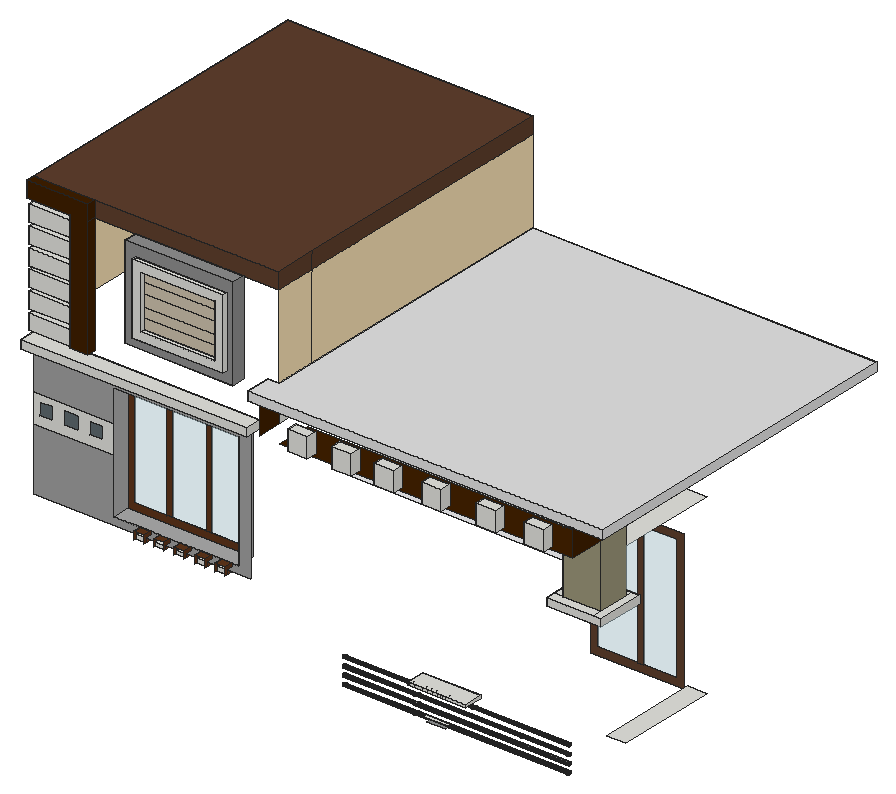
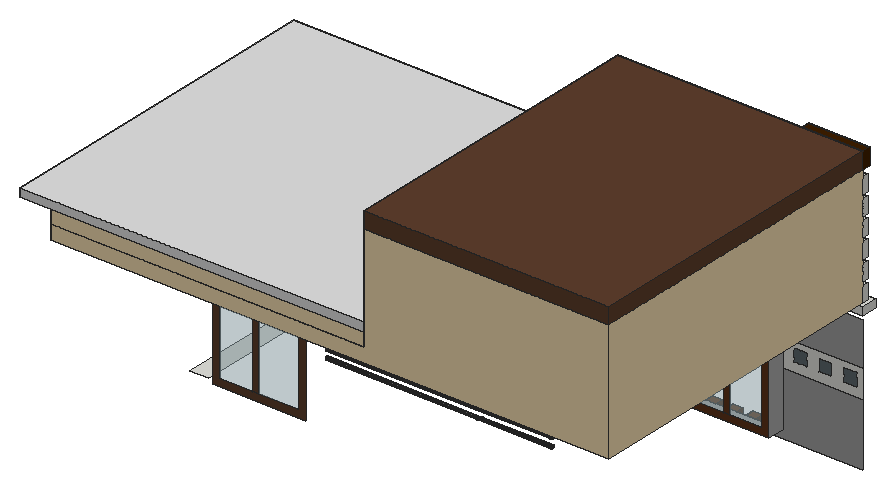
# SketchUp Ruby script. Lengths in inches.
U = 1.inch
M = Sketchup.active_model
def pt(a) = Geom::Point3d.new(a.map { |v| v * U })
def face(e, loops, mat)
  f = e.add_face(loops[0].map { |a| pt(a) })
  loops[1..].each { |l| e.add_face(l.map { |a| pt(a) }).erase! }
  f.material = f.back_material = mat if mat
  f
end
# faces: each face lists its corners as indices into pts; further lists are holes
def faces(e, pts, list, mat = nil) = list.each { |f| face(e, (f[0].is_a?(Array) ? f : [f]).map { |l| l.map { |i| pts[i] } }, mat) }
# xy, xz, yz: faces in a plane at the given z, y or x. An outline is a flat list of corners, or four numbers for a rectangle; further outlines are holes
def ring(l) = l.size == 4 ? [[l[0], l[1]], [l[2], l[1]], [l[2], l[3]], [l[0], l[3]]] : l.each_slice(2).to_a
def flat(e, list, mat, &to3) = list.each { |f| face(e, (f[0].is_a?(Array) ? f : [f]).map { |l| ring(l).map { |u, v| to3.(u, v) } }, mat) }
def xy(e, z, list, mat = nil) = flat(e, list, mat) { |x, y| [x, y, z] }
def xz(e, y, list, mat = nil) = flat(e, list, mat) { |x, z| [x, y, z] }
def yz(e, x, list, mat = nil) = flat(e, list, mat) { |y, z| [x, y, z] }
def lines(e, pts, list) = list.each { |a, b| e.add_line(pt(pts[a]), pt(pts[b])) }
# prism: a flat outline (further loops are holes) pulled along v
def prism(e, loops, v, mat = nil)
  f = face(e, loops, mat); d = Geom::Vector3d.new(v.map { |x| x * U })
  f.pushpull(f.normal.samedirection?(d) ? d.length : -d.length)
end
def box(e, o, s, mat = nil) = prism(e, [[o, [o[0] + s[0], o[1], o[2]], [o[0] + s[0], o[1] + s[1], o[2]], [o[0], o[1] + s[1], o[2]]]], [0, 0, s[2]], mat)
def at(x, y, z, deg = 0) = Geom::Transformation.translation(pt([x, y, z])) * Geom::Transformation.rotation(ORIGIN, Z_AXIS, deg.degrees)
def axes(o, x, y, z) = Geom::Transformation.new([*x, 0, *y, 0, *z, 0, *pt(o).to_a, 1])
def part(name) = M.definitions.add(name)
# library, detail: a bought-in or finely detailed component or shape, given as its bounding box
def library(name, o, s) = part(name).tap { |d| box(d.entities, o, s) }
def detail(e, o, s) = box(e.add_group.entities, o, s)
def put(e, d, t, mat = nil) = e.add_instance(d, t).tap { |i| i.material = mat if mat }
def group(e, t, mat = nil) = e.add_group.tap { |g| g.transformation = t; g.material = mat if mat }.entities
root = M.entities
M.materials.add("[0034_Wheat]").color = [245, 222, 179]
M.materials.add("[0133_Gray]").color = [128, 128, 128]
M.materials.add("[Blacktop Old 02]").color = [143, 145, 145]
M.materials.add("[Blinds Vertical Pattern]").color = [232, 232, 234]
M.materials.add("[Blinds Vertical Stripe Gray]2").color = [160, 160, 160]
M.materials.add("[Color C08]").color = [63, 31, 0]
M.materials.add("[Color M01]").color = [226, 226, 226]
M.materials.add("[Color M03]").color = [170, 170, 170]
M.materials.add("[Color M04]").color = [142, 142, 142]
M.materials.add("[Formica Speckled Grey]").color = [94, 105, 111]
M.materials.add("[Siding Rusty Metal]").color = [206, 195, 174]
M.materials.add("[Stone Coursed Rough]").color = [155, 150, 122]
M.materials.add("[Translucent Glass Safety]").color = [204, 235, 244]
M.materials["[Translucent Glass Safety]"].alpha = 0.5
M.materials.add("[Wood Cherry Original]").color = [94, 53, 26]
M.materials.add("[Wood Veneer 02]").color = [94, 63, 45]
prism(root,[[[243.46,225.17,177],[243.46,231.66,177],[243.46,231.66,178.25],[243.46,223.79,178.25],[243.46,223.79,177]]],[-24.18,0,0])
box(root,[66.16,213.82,253.05],[94.05,7.06,3.35])
box(root,[183.39,206.29,259.25],[8.18,4.44,8.19])
box(root,[281.76,206.29,259.25],[8.19,4.44,8.19])
box(root,[201.64,206.29,259.25],[8.18,4.44,8.19])
box(root,[261.82,206.29,259.25],[8.19,4.44,8.19])
box(root,[219.32,206.29,259.25],[8.19,4.44,8.19])
box(root,[239.14,206.29,259.25],[8.18,4.44,8.19])
xy(root,166.24,[[227.37,223.92,234.96,225.17]],"[Blacktop Old 02]")
xy(root,167.57,[[226.04,223.92,236.29,225.17]])
xy(root,171.3125,[[263.52,227.49,263.76,227.52,263.99,227.61,264.18,227.76,264.33,227.96,264.43,228.18,264.46,228.42,264.43,228.67,264.33,228.89,264.18,229.09,263.99,229.24,263.76,229.33,263.52,229.36,263.28,229.33,263.05,229.24,262.86,229.09,262.71,228.89,262.61,228.67,262.58,228.42,262.61,228.18,262.71,227.96,262.86,227.76,263.05,227.61,263.28,227.52]])
xy(root,171.43,[[203.52,227.49,203.76,227.52,203.99,227.61,204.18,227.76,204.29,227.9,202.75,227.9,202.86,227.76,203.05,227.61,203.28,227.52],[202.75,227.9,204.29,227.9,204.33,227.96,204.43,228.18,204.46,228.42,204.43,228.67,204.33,228.89,204.18,229.09,204.1,229.15,202.94,229.15,202.86,229.09,202.71,228.89,202.61,228.67,202.58,228.42,202.61,228.18,202.71,227.96],[202.94,229.15,204.1,229.15,203.99,229.24,203.76,229.33,203.52,229.36,203.28,229.33,203.05,229.24]])
xy(root,177,[[290.82,238.17,298.6,280.2]])
xy(root,195.78,[[110.6,218.15,114.76,220.88],[118.6,218.375,122.76,220.88],[127.16,218.375,131.32,220.88],[135.85,218.375,140.01,220.88],[144.35,218.375,148.51,220.88]],"[Wood Cherry Original]")
xy(root,197.57,[[110.6,218.15,114.76,220.88],[118.6,218.375,122.76,220.88],[127.16,218.375,131.32,220.88],[135.85,218.375,140.01,220.88],[144.35,218.375,148.51,220.88]])
xy(root,199.07,[[99.41,220.88,151.47,228.13]],"[Color M03]")
xy(root,199.07,[[110.6,217.51,114.76,220.88],[118.6,217.51,122.76,220.88],[127.16,217.51,131.32,220.88],[135.85,217.51,140.01,220.88],[144.35,217.51,148.51,220.88]],"[Wood Cherry Original]")
xy(root,228.8125,[[279.22,221.17,298.6,225.17],[298.6,221.17,301.97,241.23],[279.22,225.17,283.04,241.23],[283.04,225.17,298.6,238.17],[283.04,238.17,298.6,241.23]])
xy(root,231.84,[[279.22,221.17,298.6,225.17],[298.6,221.17,301.97,241.23],[279.22,225.17,283.04,241.23],[283.04,225.17,298.6,238.17],[283.04,238.17,298.6,241.23]])
xy(root,245.5,[[189.02,225.17,283.04,238.17]],"[Blinds Vertical Pattern]")
xy(root,246.88,[[99.41,220.88,151.47,228.13]],"[Color M03]")
xy(root,250.375,[[189.02,238.17,298.6,280.2]])
xy(root,257.875,[[283.04,225.17,298.6,238.17]])
xy(root,257.875,[[176.75,210.73,298.6,225.17]],"[Color C08]")
xy(root,263.875,[[168.19,238.17,298.6,352.92]])
xy(root,264.49,[[66.16,218.38,84.125,220.88]])
xy(root,269.1875,[[108.42,215.57,153.36,220.88]],"[Color M04]")
xy(root,269.25,[[163.51,210.73,168.19,220.88],[168.19,210.73,298.6,352.92],[298.6,210.73,311.1,352.92]])
xy(root,272.55,[[66.16,218.38,84.125,220.88]])
xy(root,272.9375,[[163.51,210.73,311.1,210.73,311.1,352.92,168.19,352.92,168.19,220.88,163.51,220.88]],"[Color M01]")
xy(root,273.55,[[112.8,213.76,150.62,215.57]])
xy(root,277.01,[[116.26,213.76,147.16,215.57]])
xy(root,280.61,[[66.16,218.38,84.125,220.88]])
xy(root,288.67,[[66.16,218.38,84.125,220.88]])
xy(root,296.74,[[66.16,218.38,84.125,220.88]])
xy(root,299.28,[[116.26,213.76,147.16,215.57]])
xy(root,302.74,[[112.8,213.76,150.62,215.57]])
xy(root,304.97,[[66.16,218.38,84.125,220.88]])
xy(root,307.625,[[66.16,217.32,84.125,220.88]])
xy(root,307.625,[[108.42,215.57,153.36,220.88]],"[Color M04]")
xy(root,314.5,[[66.16,217.32,91.59,220.88]],"[Color C08]")
xy(root,314.5,[[66.16,220.88,168.19,352.92]],"[Wood Veneer 02]")
xz(root,210.73,[[163.51,269.25,311.1,272.9375]],"[Color M01]")
xz(root,213.76,[[[112.8,273.55,150.62,302.74],[116.26,277.01,147.16,299.28]]])
xz(root,215.57,[[[112.8,273.55,150.62,302.74],[116.26,277.01,147.16,299.28]]])
xz(root,215.57,[[[108.42,269.1875,153.36,307.625],[112.8,273.55,150.62,302.74]]],"[Color M04]")
xz(root,215.57,[[116.26,277.01,147.16,281.22],[116.26,281.22,147.16,285.4375],[116.26,285.4375,147.16,290.39],[116.26,290.39,147.16,294.66],[116.26,294.66,147.16,299.28]],"[Siding Rusty Metal]")
xz(root,217.32,[[84.125,258.01,91.59,258.0625,91.59,314.5,66.16,314.5,66.16,307.625,84.125,307.625]],"[Color C08]")
xz(root,218.15,[[110.6,195.78,114.76,197.57]])
xz(root,218.375,[[118.6,195.78,122.76,197.57],[127.16,195.78,131.32,197.57],[135.85,195.78,140.01,197.57],[144.35,195.78,148.51,197.57]])
xz(root,218.38,[[66.16,257.875,84.125,258.01,84.125,264.49,66.16,264.49],[66.16,265.9375,84.125,266.07,84.125,272.55,66.16,272.55],[66.16,274,84.125,274.13,84.125,280.61,66.16,280.61],[66.16,282.0625,84.125,282.19,84.125,288.67,66.16,288.67],[66.16,290.125,84.125,290.26,84.125,296.74,66.16,296.74],
  [66.16,298.36,84.125,298.49,84.125,304.97,66.16,304.97]])
xz(root,220.88,[[110.6,197.57,114.76,199.07],[118.6,197.57,122.76,199.07],[127.16,197.57,131.32,199.07],[135.85,197.57,140.01,199.07],[144.35,197.57,148.51,199.07],
  [[66.16,221.98,99.41,233.67],[68.73,225.92,73.98,231.17],[89.61,225.92,94.86,231.17],[79.11,225.92,84.36,231.17]],[66.16,257.875,66.16,264.49,84.125,264.49,84.125,258.01],[84.125,258.01,84.125,307.625,66.16,307.625,66.16,314.5,91.59,314.5,91.59,258.0625],[66.16,265.9375,66.16,272.55,84.125,272.55,84.125,266.07],[108.42,269.1875,153.36,307.625],
  [163.51,269.25,168.19,272.9375],[66.16,274,66.16,280.61,84.125,280.61,84.125,274.13],[66.16,282.0625,66.16,288.67,84.125,288.67,84.125,282.19],[66.16,290.125,66.16,296.74,84.125,296.74,84.125,290.26],[66.16,298.36,66.16,304.97,84.125,304.97,84.125,298.49]])
xz(root,220.88,[[66.16,195.78,156.36,195.78,156.36,251.53,66.16,251.53,66.16,233.67,99.41,233.67,99.41,246.88,151.47,246.88,151.47,199.07,148.51,199.07,148.51,197.57,144.35,197.57,144.35,199.07,140.01,199.07,140.01,197.57,135.85,197.57,135.85,199.07,131.32,199.07,131.32,197.57,127.16,197.57,127.16,199.07,122.76,199.07,122.76,197.57,118.6,197.57,118.6,199.07,114.76,199.07,114.76,197.57,110.6,197.57,110.6,199.07,99.41,199.07,99.41,221.98,66.16,221.98]],"[Blinds Vertical Stripe Gray]2")
xz(root,220.88,[[66.16,264.49,84.125,264.49,84.125,266.07,66.16,265.9375],[66.16,272.55,84.125,272.55,84.125,274.13,66.16,274],[66.16,280.61,84.125,280.61,84.125,282.19,66.16,282.0625],[66.16,288.67,84.125,288.67,84.125,290.26,66.16,290.125],[66.16,296.74,84.125,296.74,84.125,298.49,66.16,298.36],
  [66.16,304.97,84.125,307.625]],"[Color C08]")
xz(root,220.88,[[68.73,225.92,73.98,231.17],[79.11,225.92,84.36,231.17],[89.61,225.92,94.86,231.17]],"[Formica Speckled Grey]")
xz(root,220.88,[[91.59,307.625,168.19,314.5]],"[Wood Veneer 02]")
xz(root,221.17,[[279.22,228.8125,301.97,231.84]])
xz(root,225.17,[[283.04,231.84,298.6,257.875]],"[Stone Coursed Rough]")
xz(root,228.13,[[102.28,201.94,115.85,244.01],[118.18,201.94,132.16,244.01],[134.49,201.94,148.6,244.01]],"[Translucent Glass Safety]")
xz(root,228.13,[[[99.41,199.07,151.47,246.88],[102.28,201.94,148.6,244.01]],[115.85,201.94,118.18,244.01],[132.16,201.94,134.49,244.01]],"[Wood Cherry Original]")
xz(root,238.17,[[189.02,245.5,283.04,250.375],[189.02,250.375,283.04,257.875],[283.04,250.375,298.6,257.875],[168.19,257.875,298.6,263.875]])
xz(root,238.17,[[283.04,231.84,298.6,250.375]],"[Stone Coursed Rough]")
xz(root,241.23,[[279.22,228.8125,301.97,231.84]])
xz(root,280.2,[[253.41,178.34,269.83,230.1],[272.58,178.34,286.12,230.1]],"[Translucent Glass Safety]")
xz(root,280.2,[[[250.45,175.375,289.08,233.0625],[253.41,178.34,286.12,230.1]],[269.83,178.34,272.58,230.1]],"[Wood Veneer 02]")
xz(root,352.92,[[66.16,257.875,66.16,307.625,168.19,307.625,168.19,263.875,298.6,263.875,298.6,257.875],[168.19,263.875,298.6,269.25]],"[0034_Wheat]")
xz(root,352.92,[[168.19,269.25,311.1,272.9375]],"[Color M01]")
xz(root,352.92,[[66.16,307.625,168.19,314.5]],"[Wood Veneer 02]")
yz(root,66.16,[[218.38,257.875,220.88,264.49],[218.38,265.9375,220.88,272.55],[218.38,274,220.88,280.61],[218.38,282.0625,220.88,288.67],[218.38,290.125,220.88,296.74],
  [218.38,298.36,220.88,304.97]])
yz(root,66.16,[[220.88,257.875,352.92,307.625]],"[0034_Wheat]")
yz(root,66.16,[[217.32,307.625,220.88,314.5]],"[Color C08]")
yz(root,66.16,[[220.88,307.625,352.92,314.5]],"[Wood Veneer 02]")
yz(root,84.125,[[218.38,258.01,220.88,264.49],[218.38,266.07,220.88,272.55],[218.38,274.13,220.88,280.61],[218.38,282.19,220.88,288.67],[218.38,290.26,220.88,296.74],
  [218.38,298.49,220.88,304.97]])
yz(root,84.125,[[217.32,258.01,218.38,264.49],[217.32,264.49,220.88,266.07],[217.32,266.07,218.38,272.55],[217.32,272.55,220.88,274.13],[217.32,274.13,218.38,280.61],
  [217.32,280.61,220.88,282.19],[217.32,282.19,218.38,288.67],[217.32,288.67,220.88,290.26],[217.32,290.26,218.38,296.74],[217.32,296.74,220.88,298.49],
  [217.32,298.49,218.38,304.97],[217.32,304.97,220.88,307.625]],"[Color C08]")
yz(root,91.59,[[217.32,258.0625,220.88,307.625],[217.32,307.625,220.88,314.5]],"[Color C08]")
yz(root,99.41,[[220.88,199.07,228.13,246.88]],"[Color M03]")
yz(root,108.42,[[215.57,269.1875,220.88,307.625]],"[Color M04]")
yz(root,110.6,[[217.51,195.78,217.51,199.07,220.88,199.07,220.88,197.57,218.15,197.57,218.15,195.78]],"[Wood Cherry Original]")
yz(root,112.8,[[213.76,273.55,215.57,302.74]])
yz(root,114.76,[[217.51,195.78,218.15,195.78,218.15,197.57,220.88,197.57,220.88,199.07,217.51,199.07]],"[Wood Cherry Original]")
yz(root,116.26,[[213.76,277.01,215.57,299.28]])
yz(root,118.6,[[217.51,195.78,217.51,199.07,220.88,199.07,220.88,197.57,218.375,197.57,218.375,195.78]],"[Wood Cherry Original]")
yz(root,122.76,[[217.51,195.78,218.375,195.78,218.375,197.57,220.88,197.57,220.88,199.07,217.51,199.07]],"[Wood Cherry Original]")
yz(root,127.16,[[217.51,195.78,217.51,199.07,220.88,199.07,220.88,197.57,218.375,197.57,218.375,195.78]],"[Wood Cherry Original]")
yz(root,131.32,[[217.51,195.78,218.375,195.78,218.375,197.57,220.88,197.57,220.88,199.07,217.51,199.07]],"[Wood Cherry Original]")
yz(root,135.85,[[217.51,195.78,217.51,199.07,220.88,199.07,220.88,197.57,218.375,197.57,218.375,195.78]],"[Wood Cherry Original]")
yz(root,140.01,[[217.51,195.78,218.375,195.78,218.375,197.57,220.88,197.57,220.88,199.07,217.51,199.07]],"[Wood Cherry Original]")
yz(root,144.35,[[217.51,195.78,217.51,199.07,220.88,199.07,220.88,197.57,218.375,197.57,218.375,195.78]],"[Wood Cherry Original]")
yz(root,147.16,[[213.76,277.01,215.57,299.28]])
yz(root,148.51,[[217.51,195.78,218.375,195.78,218.375,197.57,220.88,197.57,220.88,199.07,217.51,199.07]],"[Wood Cherry Original]")
yz(root,150.62,[[213.76,273.55,215.57,302.74]])
yz(root,151.47,[[220.88,199.07,228.13,246.88]],"[Color M03]")
yz(root,153.36,[[215.57,269.1875,220.88,307.625]],"[Color M04]")
yz(root,163.51,[[210.73,269.25,220.88,272.9375]])
yz(root,168.19,[[220.88,257.875,238.17,269.25],[238.17,263.875,352.92,269.25],[220.88,269.25,238.17,272.9375],[238.17,269.25,352.92,272.9375]])
yz(root,168.19,[[220.88,272.9375,238.17,307.625],[238.17,272.9375,352.92,307.625]],"[0034_Wheat]")
yz(root,168.19,[[210.73,257.875,220.88,269.25]],"[Color C08]")
yz(root,168.19,[[220.88,307.625,238.17,314.5],[238.17,307.625,352.92,314.5]],"[Wood Veneer 02]")
yz(root,219.28,[[228.53,163.93,228.6875,163.95,228.84,164.02,228.97,164.12,229.07,164.24,229.13,164.4,229.15,164.56,229.13,164.72,229.07,164.87,228.97,165,228.84,165.1,228.6875,165.16,228.53,165.18,228.36,165.16,228.21,165.1,228.08,165,227.98,164.87,227.92,164.72,227.9,164.56,227.92,164.4,227.98,164.24,228.08,164.12,228.21,164.02,228.36,163.95],[228.53,167.43,228.6875,167.45,228.84,167.52,228.97,167.62,229.07,167.74,229.13,167.9,229.15,168.06,229.13,168.22,229.07,168.37,228.97,168.5,228.84,168.6,228.6875,168.66,228.53,168.68,228.36,168.66,228.21,168.6,228.08,168.5,227.98,168.37,227.92,168.22,227.9,168.06,227.92,167.9,227.98,167.74,228.08,167.62,228.21,167.52,228.36,167.45],[228.53,170.81,228.6875,170.83,228.84,170.89,228.97,170.99,229.07,171.12,229.13,171.27,229.15,171.43,229.13,171.59,229.07,171.74,228.97,171.875,228.84,171.97,228.6875,172.04,228.53,172.06,228.36,172.04,228.21,171.97,228.08,171.875,227.98,171.74,227.92,171.59,227.9,171.43,227.92,171.27,227.98,171.12,228.08,170.99,228.21,170.89,228.36,170.83]])
yz(root,219.47,[[228.53,167.43,228.6875,167.45,228.84,167.52,228.97,167.62,229.07,167.74,229.13,167.9,229.15,168.06,229.13,168.22,229.07,168.37,228.97,168.5,228.84,168.6,228.6875,168.66,228.53,168.68,228.36,168.66,228.21,168.6,228.08,168.5,227.98,168.37,227.92,168.22,227.9,168.06,227.92,167.9,227.98,167.74,228.08,167.62,228.21,167.52,228.36,167.45]])
yz(root,243.46,[[228.44,174.54,228.3,174.5625,228.16,174.62,228.04,174.71,227.95,174.83,227.9,174.96,227.88,175.11,227.9,175.25,227.95,175.39,228.04,175.5,228.16,175.59,228.3,175.65,228.44,175.67,228.59,175.65,228.72,175.59,228.84,175.5,228.93,175.39,228.98,175.25,229,175.11,228.98,174.96,228.93,174.83,228.84,174.71,228.72,174.62,228.59,174.5625]])
yz(root,279.22,[[221.17,228.8125,241.23,231.84]])
yz(root,283.04,[[225.17,245.5,238.17,257.875]])
yz(root,283.04,[[225.17,231.84,238.17,245.5]],"[Stone Coursed Rough]")
yz(root,298.6,[[210.73,257.875,238.17,257.875,238.17,263.875,352.92,263.875,352.92,269.25,210.73,269.25],[238.17,257.875,352.92,263.875]],"[Color C08]")
yz(root,298.6,[[225.17,231.84,238.17,257.875]],"[Stone Coursed Rough]")
yz(root,301.97,[[221.17,228.8125,241.23,231.84]])
yz(root,311.1,[[210.73,269.25,352.92,272.9375]],"[Color M01]")
p = [[219.28,228.53,163.93],[219.28,228.36,163.95],[189.02,228.36,163.95],[189.02,228.53,163.93],[283.04,228.53,163.93],[283.04,228.36,163.95],
  [219.28,228.6875,163.95],[189.02,228.6875,163.95],[283.04,228.6875,163.95],[219.28,228.21,164.02],[219.28,228.08,164.12],[189.02,228.08,164.12],
  [189.02,228.21,164.02],[283.04,228.21,164.02],[283.04,228.08,164.12],[219.28,228.84,164.02],[189.02,228.84,164.02],[283.04,228.84,164.02],
  [219.28,228.97,164.12],[189.02,228.97,164.12],[283.04,228.97,164.12],[219.28,227.98,164.24],[189.02,227.98,164.24],[283.04,227.98,164.24],
  [219.28,229.07,164.24],[189.02,229.07,164.24],[283.04,229.07,164.24],[219.28,227.92,164.4],[189.02,227.92,164.4],[283.04,227.92,164.4],
  [219.28,229.13,164.4],[189.02,229.13,164.4],[283.04,229.13,164.4],[219.28,227.9,164.56],[189.02,227.9,164.56],[283.04,227.9,164.56],
  [219.28,229.15,164.56],[189.02,229.15,164.56],[283.04,229.15,164.56],[219.28,227.92,164.72],[189.02,227.92,164.72],[283.04,227.92,164.72],
  [219.28,229.13,164.72],[189.02,229.13,164.72],[283.04,229.13,164.72],[219.28,227.98,164.87],[189.02,227.98,164.87],[283.04,227.98,164.87],
  [219.28,229.07,164.87],[189.02,229.07,164.87],[283.04,229.07,164.87],[219.28,228.08,165],[189.02,228.08,165],[283.04,228.08,165],
  [219.28,228.97,165],[189.02,228.97,165],[283.04,228.97,165],[219.28,228.21,165.1],[189.02,228.21,165.1],[283.04,228.21,165.1],
  [219.28,228.84,165.1],[189.02,228.84,165.1],[283.04,228.84,165.1],[219.28,228.36,165.16],[189.02,228.36,165.16],[283.04,228.36,165.16],
  [219.28,228.6875,165.16],[189.02,228.6875,165.16],[283.04,228.6875,165.16],[219.28,228.53,165.18],[189.02,228.53,165.18],[283.04,228.53,165.18],
  [219.28,228.53,167.43],[219.28,228.36,167.45],[189.02,228.36,167.45],[189.02,228.53,167.43],[219.47,228.53,167.43],[219.47,228.36,167.45],
  [283.04,228.36,167.45],[283.04,228.53,167.43],[219.28,228.6875,167.45],[189.02,228.6875,167.45],[219.47,228.6875,167.45],[283.04,228.6875,167.45],
  [219.28,228.21,167.52],[219.28,228.08,167.62],[189.02,228.08,167.62],[189.02,228.21,167.52],[219.47,228.21,167.52],[219.47,228.08,167.62],
  [283.04,228.08,167.62],[283.04,228.21,167.52],[219.28,228.84,167.52],[189.02,228.84,167.52],[219.47,228.84,167.52],[283.04,228.84,167.52],
  [219.28,228.97,167.62],[189.02,228.97,167.62],[219.47,228.97,167.62],[283.04,228.97,167.62],[219.28,227.98,167.74],[189.02,227.98,167.74],
  [219.47,227.98,167.74],[283.04,227.98,167.74],[219.28,229.07,167.74],[189.02,229.07,167.74],[219.47,229.07,167.74],[283.04,229.07,167.74],
  [219.28,227.92,167.9],[189.02,227.92,167.9],[219.47,227.92,167.9],[283.04,227.92,167.9],[219.28,229.13,167.9],[189.02,229.13,167.9],
  [219.47,229.13,167.9],[283.04,229.13,167.9],[219.28,227.9,168.06],[189.02,227.9,168.06],[219.47,227.9,168.06],[283.04,227.9,168.06],
  [219.28,229.15,168.06],[189.02,229.15,168.06],[219.47,229.15,168.06],[283.04,229.15,168.06],[219.28,227.92,168.22],[189.02,227.92,168.22],
  [219.47,227.92,168.22],[283.04,227.92,168.22],[219.28,229.13,168.22],[189.02,229.13,168.22],[219.47,229.13,168.22],[283.04,229.13,168.22],
  [219.28,227.98,168.37],[189.02,227.98,168.37],[219.47,227.98,168.37],[283.04,227.98,168.37],[219.28,229.07,168.37],[189.02,229.07,168.37],
  [219.47,229.07,168.37],[283.04,229.07,168.37],[219.28,228.08,168.5],[189.02,228.08,168.5],[219.47,228.08,168.5],[283.04,228.08,168.5],
  [219.28,228.97,168.5],[189.02,228.97,168.5],[219.47,228.97,168.5],[283.04,228.97,168.5],[219.28,228.21,168.6],[189.02,228.21,168.6],
  [219.47,228.21,168.6],[283.04,228.21,168.6],[219.28,228.84,168.6],[189.02,228.84,168.6],[219.47,228.84,168.6],[283.04,228.84,168.6],
  [219.28,228.36,168.66],[189.02,228.36,168.66],[219.47,228.36,168.66],[283.04,228.36,168.66],[219.28,228.6875,168.66],[189.02,228.6875,168.66],
  [219.47,228.6875,168.66],[283.04,228.6875,168.66],[219.28,228.53,168.68],[189.02,228.53,168.68],[219.47,228.53,168.68],[283.04,228.53,168.68],
  [219.28,228.36,170.83],[219.28,228.21,170.89],[189.02,228.21,170.89],[189.02,228.36,170.83],[283.04,228.36,170.83],[283.04,228.21,170.89],
  [219.28,228.53,170.81],[189.02,228.53,170.81],[283.04,228.53,170.81],[219.28,228.6875,170.83],[189.02,228.6875,170.83],[283.04,228.6875,170.83],
  [219.28,228.84,170.89],[189.02,228.84,170.89],[283.04,228.84,170.89],[219.28,228.08,170.99],[189.02,228.08,170.99],[283.04,228.08,170.99],
  [219.28,228.97,170.99],[189.02,228.97,170.99],[283.04,228.97,170.99],[219.28,227.98,171.12],[189.02,227.98,171.12],[283.04,227.98,171.12],
  [219.28,229.07,171.12],[189.02,229.07,171.12],[283.04,229.07,171.12],[219.28,227.92,171.27],[189.02,227.92,171.27],[283.04,227.92,171.27],
  [219.28,229.13,171.27],[189.02,229.13,171.27],[283.04,229.13,171.27],[219.28,227.9,171.43],[204.29,227.9,171.43],[202.75,227.9,171.43],
  [189.02,227.9,171.43],[283.04,227.9,171.43],[219.28,229.15,171.43],[189.02,229.15,171.43],[202.94,229.15,171.43],[204.1,229.15,171.43],
  [283.04,229.15,171.43],[219.28,227.92,171.59],[189.02,227.92,171.59],[283.04,227.92,171.59],[219.28,229.13,171.59],[189.02,229.13,171.59],
  [283.04,229.13,171.59],[219.28,227.98,171.74],[189.02,227.98,171.74],[283.04,227.98,171.74],[219.28,229.07,171.74],[189.02,229.07,171.74],
  [283.04,229.07,171.74],[219.28,228.08,171.875],[189.02,228.08,171.875],[283.04,228.08,171.875],[219.28,228.97,171.875],[189.02,228.97,171.875],
  [283.04,228.97,171.875],[219.28,228.21,171.97],[189.02,228.21,171.97],[283.04,228.21,171.97],[219.28,228.84,171.97],[189.02,228.84,171.97],
  [283.04,228.84,171.97],[219.28,228.36,172.04],[189.02,228.36,172.04],[283.04,228.36,172.04],[219.28,228.53,172.06],[189.02,228.53,172.06],
  [283.04,228.53,172.06],[219.28,228.6875,172.04],[189.02,228.6875,172.04],[283.04,228.6875,172.04],[243.46,228.44,174.54],[243.46,228.3,174.5625],
  [189.02,228.3,174.5625],[189.02,228.44,174.54],[283.04,228.44,174.54],[283.04,228.3,174.5625],[243.46,228.59,174.5625],[189.02,228.59,174.5625],
  [283.04,228.59,174.5625],[243.46,228.16,174.62],[243.46,228.04,174.71],[189.02,228.04,174.71],[189.02,228.16,174.62],[283.04,228.16,174.62],
  [283.04,228.04,174.71],[243.46,228.72,174.62],[189.02,228.72,174.62],[283.04,228.72,174.62],[243.46,228.84,174.71],[189.02,228.84,174.71],
  [283.04,228.84,174.71],[243.46,227.95,174.83],[189.02,227.95,174.83],[283.04,227.95,174.83],[243.46,228.93,174.83],[189.02,228.93,174.83],
  [283.04,228.93,174.83],[243.46,227.9,174.96],[189.02,227.9,174.96],[283.04,227.9,174.96],[243.46,228.98,174.96],[189.02,228.98,174.96],
  [283.04,228.98,174.96],[243.46,227.88,175.11],[189.02,227.88,175.11],[283.04,227.88,175.11],[243.46,229,175.11],[189.02,229,175.11],
  [283.04,229,175.11],[243.46,227.9,175.25],[189.02,227.9,175.25],[283.04,227.9,175.25],[243.46,228.98,175.25],[189.02,228.98,175.25],
  [283.04,228.98,175.25],[243.46,227.95,175.39],[189.02,227.95,175.39],[283.04,227.95,175.39],[243.46,228.93,175.39],[189.02,228.93,175.39],
  [283.04,228.93,175.39],[243.46,228.04,175.5],[189.02,228.04,175.5],[283.04,228.04,175.5],[243.46,228.84,175.5],[189.02,228.84,175.5],
  [283.04,228.84,175.5],[243.46,228.16,175.59],[189.02,228.16,175.59],[283.04,228.16,175.59],[243.46,228.72,175.59],[189.02,228.72,175.59],
  [283.04,228.72,175.59],[243.46,228.3,175.65],[189.02,228.3,175.65],[283.04,228.3,175.65],[243.46,228.44,175.67],[189.02,228.44,175.67],
  [283.04,228.44,175.67],[243.46,228.59,175.65],[189.02,228.59,175.65],[283.04,228.59,175.65],[66.16,220.88,257.875],[84.125,220.88,258.01],
  [84.125,218.38,258.01],[66.16,218.38,257.875],[91.59,220.88,258.0625],[91.59,217.32,258.0625],[84.125,217.32,258.01],[66.16,220.88,265.9375],
  [84.125,220.88,266.07],[84.125,218.38,266.07],[66.16,218.38,265.9375],[66.16,220.88,274],[84.125,220.88,274.13],[84.125,218.38,274.13],
  [66.16,218.38,274],[66.16,220.88,282.0625],[84.125,220.88,282.19],[84.125,218.38,282.19],[66.16,218.38,282.0625],[66.16,220.88,290.125],
  [84.125,220.88,290.26],[84.125,218.38,290.26],[66.16,218.38,290.125],[66.16,220.88,298.36],[84.125,220.88,298.49],[84.125,218.38,298.49],
  [66.16,218.38,298.36]]
faces(root,p,[[0,1,2,3],[1,0,4,5],[6,0,3,7],[0,6,8,4],[9,10,11,12],[10,9,13,14],[1,9,12,2],[9,1,5,13],
  [15,6,7,16],[6,15,17,8],[18,15,16,19],[15,18,20,17],[10,21,22,11],[21,10,14,23],[24,18,19,25],[18,24,26,20],
  [21,27,28,22],[27,21,23,29],[30,24,25,31],[24,30,32,26],[27,33,34,28],[33,27,29,35],[36,30,31,37],[30,36,38,32],
  [33,39,40,34],[39,33,35,41],[42,36,37,43],[36,42,44,38],[39,45,46,40],[45,39,41,47],[48,42,43,49],[42,48,50,44],
  [45,51,52,46],[51,45,47,53],[54,48,49,55],[48,54,56,50],[51,57,58,52],[57,51,53,59],[60,54,55,61],[54,60,62,56],
  [57,63,64,58],[63,57,59,65],[66,60,61,67],[60,66,68,62],[63,69,70,64],[69,63,65,71],[69,66,67,70],[66,69,71,68],
  [72,73,74,75],[78,77,76,79],[80,72,75,81],[79,76,82,83],[84,85,86,87],[90,89,88,91],[73,84,87,74],[91,88,77,78],
  [92,80,81,93],[83,82,94,95],[96,92,93,97],[95,94,98,99],[85,100,101,86],[103,102,89,90],[104,96,97,105],[99,98,106,107],
  [100,108,109,101],[111,110,102,103],[112,104,105,113],[107,106,114,115],[108,116,117,109],[119,118,110,111],[120,112,113,121],[115,114,122,123],
  [116,124,125,117],[127,126,118,119],[128,120,121,129],[123,122,130,131],[124,132,133,125],[135,134,126,127],[136,128,129,137],[131,130,138,139],
  [132,140,141,133],[143,142,134,135],[144,136,137,145],[139,138,146,147],[140,148,149,141],[151,150,142,143],[152,144,145,153],[147,146,154,155],
  [148,156,157,149],[159,158,150,151],[160,152,153,161],[155,154,162,163],[156,164,165,157],[167,166,158,159],[164,160,161,165],[163,162,166,167],
  [168,169,170,171],[169,168,172,173],[174,168,171,175],[168,174,176,172],[177,174,175,178],[174,177,179,176],[180,177,178,181],[177,180,182,179],
  [169,183,184,170],[183,169,173,185],[186,180,181,187],[180,186,188,182],[183,189,190,184],[189,183,185,191],[192,186,187,193],[186,192,194,188],
  [189,195,196,190],[195,189,191,197],[198,192,193,199],[192,198,200,194],[195,201,202,203,204,196],[201,195,197,205],[206,198,199,207,208,209],[198,206,210,200],
  [201,211,212,204,203,202],[211,201,205,213],[214,206,209,208,207,215],[206,214,216,210],[211,217,218,212],[217,211,213,219],[220,214,215,221],[214,220,222,216],
  [217,223,224,218],[223,217,219,225],[226,220,221,227],[220,226,228,222],[223,229,230,224],[229,223,225,231],[232,226,227,233],[226,232,234,228],
  [229,235,236,230],[235,229,231,237],[235,238,239,236],[238,235,237,240],[238,241,242,239],[241,238,240,243],[241,232,233,242],[232,241,243,234],
  [244,245,246,247],[245,244,248,249],[250,244,247,251],[244,250,252,248],[253,254,255,256],[254,253,257,258],[245,253,256,246],[253,245,249,257],
  [259,250,251,260],[250,259,261,252],[262,259,260,263],[259,262,264,261],[254,265,266,255],[265,254,258,267],[268,262,263,269],[262,268,270,264],
  [265,271,272,266],[271,265,267,273],[274,268,269,275],[268,274,276,270],[271,277,278,272],[277,271,273,279],[280,274,275,281],[274,280,282,276],
  [277,283,284,278],[283,277,279,285],[286,280,281,287],[280,286,288,282],[283,289,290,284],[289,283,285,291],[292,286,287,293],[286,292,294,288],
  [289,295,296,290],[295,289,291,297],[298,292,293,299],[292,298,300,294],[295,301,302,296],[301,295,297,303],[304,298,299,305],[298,304,306,300],
  [301,307,308,302],[307,301,303,309],[307,310,311,308],[310,307,309,312],[310,313,314,311],[313,310,312,315],[313,304,305,314],[304,313,315,306]],"[0133_Gray]")
faces(root,p,[[73,72,76,77],[72,80,82,76],[85,84,88,89],[84,73,77,88],[80,92,94,82],[92,96,98,94],[100,85,89,102],[96,104,106,98],
  [108,100,102,110],[104,112,114,106],[116,108,110,118],[112,120,122,114],[124,116,118,126],[120,128,130,122],[132,124,126,134],[128,136,138,130],
  [140,132,134,142],[136,144,146,138],[148,140,142,150],[144,152,154,146],[156,148,150,158],[152,160,162,154],[164,156,158,166],[160,164,166,162],
  [316,317,318,319],[317,320,321,322,318],[323,324,325,326],[327,328,329,330],[331,332,333,334],[335,336,337,338],[339,340,341,342]])
